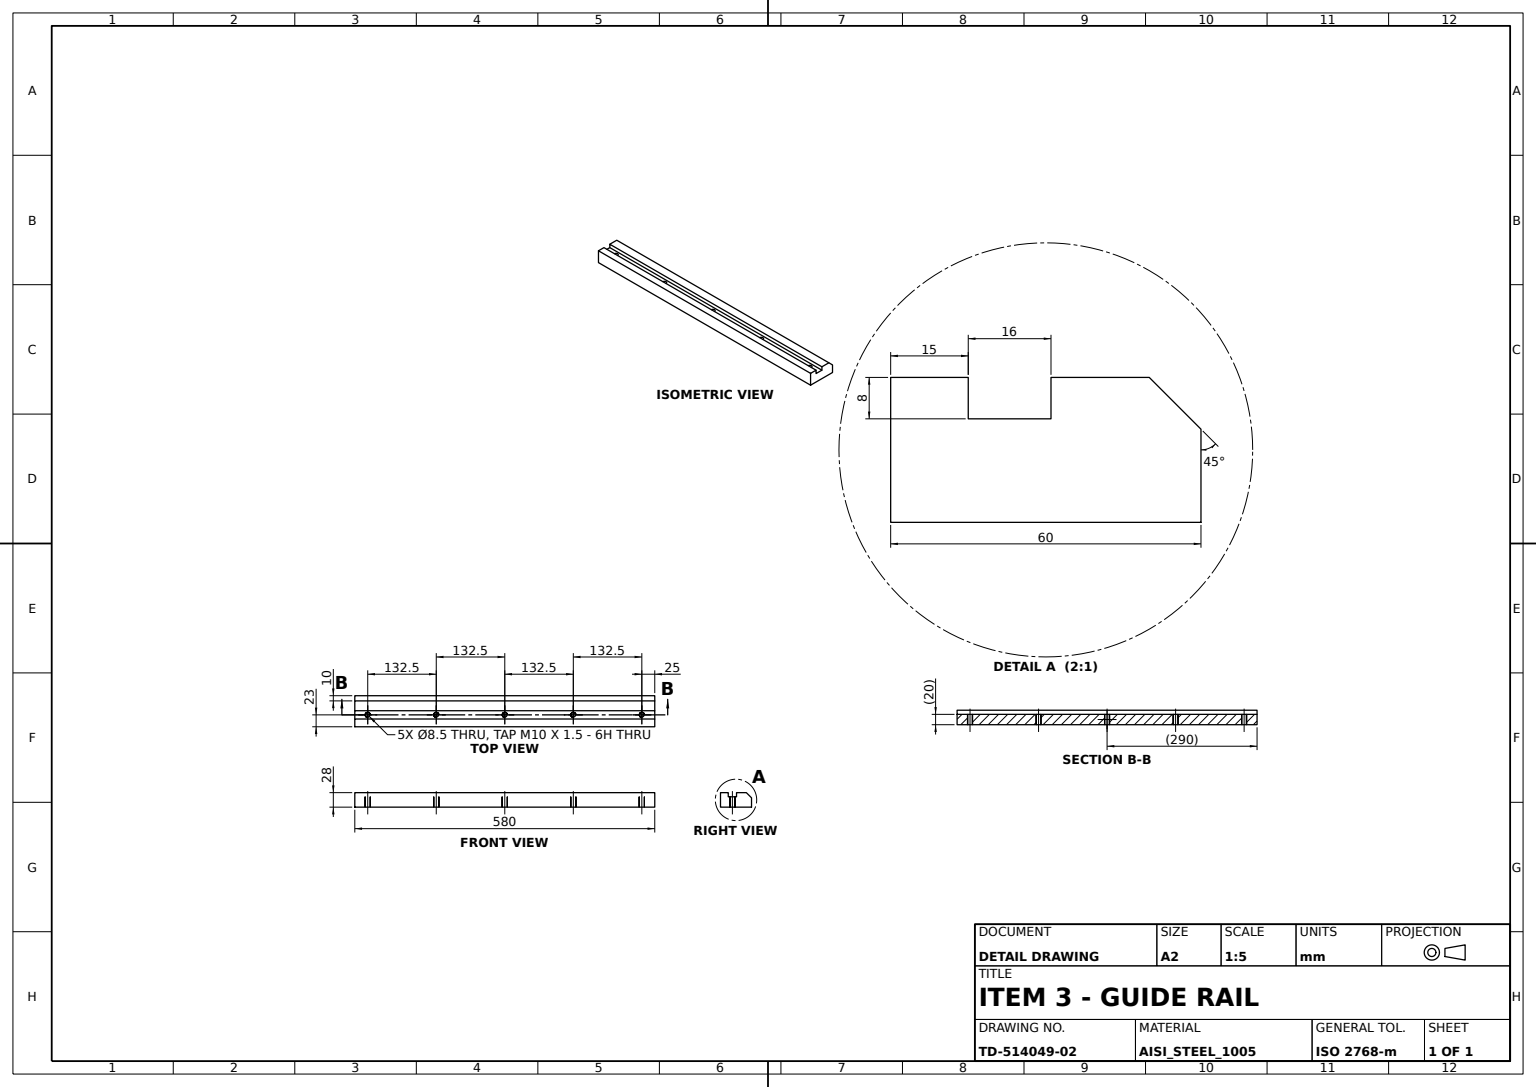
ISO-10303-21;
HEADER;
FILE_DESCRIPTION((''),'2;1');
FILE_NAME('','',(''),(''),'','','');
FILE_SCHEMA(('AUTOMOTIVE_DESIGN'));
ENDSEC;
DATA;
#1=APPLICATION_CONTEXT('');
#2=PRODUCT_CONTEXT('',#1,'mechanical');
#3=PRODUCT('','','',(#2));
#4=PRODUCT_DEFINITION_FORMATION('','',#3);
#5=PRODUCT_DEFINITION_CONTEXT('',#1,'design');
#6=PRODUCT_DEFINITION('','',#4,#5);
#7=PRODUCT_DEFINITION_SHAPE('','',#6);
#8=(LENGTH_UNIT()NAMED_UNIT(*)SI_UNIT(.MILLI.,.METRE.));
#9=(NAMED_UNIT(*)PLANE_ANGLE_UNIT()SI_UNIT($,.RADIAN.));
#10=(NAMED_UNIT(*)SI_UNIT($,.STERADIAN.)SOLID_ANGLE_UNIT());
#11=UNCERTAINTY_MEASURE_WITH_UNIT(LENGTH_MEASURE(0.005),#8,'distance_accuracy_value','');
#12=(GEOMETRIC_REPRESENTATION_CONTEXT(3)GLOBAL_UNCERTAINTY_ASSIGNED_CONTEXT((#11))GLOBAL_UNIT_ASSIGNED_CONTEXT((#8,#9,#10))REPRESENTATION_CONTEXT('',''));
#13=CARTESIAN_POINT('',(0.,32.75,265.));
#14=VERTEX_POINT('',#13);
#15=CARTESIAN_POINT('',(0.,37.,265.));
#16=DIRECTION('',(-1.,0.,0.));
#17=DIRECTION('',(0.,-1.,0.));
#18=AXIS2_PLACEMENT_3D('',#15,#16,#17);
#19=CIRCLE('',#18,4.25);
#20=EDGE_CURVE('',#14,#14,#19,.T.);
#21=ORIENTED_EDGE('',*,*,#20,.F.);
#22=EDGE_LOOP('',(#21));
#23=FACE_BOUND('',#22,.T.);
#24=CARTESIAN_POINT('',(-20.,41.25,265.));
#25=VERTEX_POINT('',#24);
#26=CARTESIAN_POINT('',(-20.,37.,265.));
#27=DIRECTION('',(1.,0.,0.));
#28=DIRECTION('',(0.,1.,0.));
#29=AXIS2_PLACEMENT_3D('',#26,#27,#28);
#30=CIRCLE('',#29,4.25);
#31=EDGE_CURVE('',#25,#25,#30,.T.);
#32=ORIENTED_EDGE('',*,*,#31,.F.);
#33=EDGE_LOOP('',(#32));
#34=FACE_BOUND('',#33,.T.);
#35=CYLINDRICAL_SURFACE('',#29,4.25);
#36=ADVANCED_FACE('',(#23,#34),#35,.F.);
#37=CARTESIAN_POINT('',(-20.,41.25,-132.5));
#38=VERTEX_POINT('',#37);
#39=CARTESIAN_POINT('',(-20.,37.,-132.5));
#40=AXIS2_PLACEMENT_3D('',#39,#27,#28);
#41=CIRCLE('',#40,4.25);
#42=EDGE_CURVE('',#38,#38,#41,.T.);
#43=ORIENTED_EDGE('',*,*,#42,.F.);
#44=EDGE_LOOP('',(#43));
#45=FACE_BOUND('',#44,.T.);
#46=CARTESIAN_POINT('',(0.,32.75,-132.5));
#47=VERTEX_POINT('',#46);
#48=CARTESIAN_POINT('',(0.,37.,-132.5));
#49=AXIS2_PLACEMENT_3D('',#48,#16,#17);
#50=CIRCLE('',#49,4.25);
#51=EDGE_CURVE('',#47,#47,#50,.T.);
#52=ORIENTED_EDGE('',*,*,#51,.F.);
#53=EDGE_LOOP('',(#52));
#54=FACE_BOUND('',#53,.T.);
#55=CYLINDRICAL_SURFACE('',#40,4.25);
#56=ADVANCED_FACE('',(#45,#54),#55,.F.);
#57=CARTESIAN_POINT('',(0.,60.,290.));
#58=VERTEX_POINT('',#57);
#59=CARTESIAN_POINT('',(-28.,60.,290.));
#60=VERTEX_POINT('',#59);
#61=VECTOR('',#16,1000.);
#62=LINE('',#57,#61);
#63=EDGE_CURVE('',#58,#60,#62,.T.);
#64=ORIENTED_EDGE('',*,*,#63,.F.);
#65=CARTESIAN_POINT('',(0.,60.,-290.));
#66=VERTEX_POINT('',#65);
#67=DIRECTION('',(0.,0.,-1.));
#68=VECTOR('',#67,1000.);
#69=LINE('',#57,#68);
#70=EDGE_CURVE('',#58,#66,#69,.T.);
#71=ORIENTED_EDGE('',*,*,#70,.T.);
#72=CARTESIAN_POINT('',(-28.,60.,-290.));
#73=VERTEX_POINT('',#72);
#74=LINE('',#65,#61);
#75=EDGE_CURVE('',#66,#73,#74,.T.);
#76=ORIENTED_EDGE('',*,*,#75,.T.);
#77=LINE('',#59,#68);
#78=EDGE_CURVE('',#60,#73,#77,.T.);
#79=ORIENTED_EDGE('',*,*,#78,.F.);
#80=EDGE_LOOP('',(#64,#71,#76,#79));
#81=FACE_BOUND('',#80,.T.);
#82=AXIS2_PLACEMENT_3D('',#57,#17,#27);
#83=PLANE('',#82);
#84=ADVANCED_FACE('',(#81),#83,.F.);
#85=CARTESIAN_POINT('',(-20.,29.,-290.));
#86=VERTEX_POINT('',#85);
#87=CARTESIAN_POINT('',(-28.,29.,-290.));
#88=VERTEX_POINT('',#87);
#89=LINE('',#85,#61);
#90=EDGE_CURVE('',#86,#88,#89,.T.);
#91=ORIENTED_EDGE('',*,*,#90,.T.);
#92=CARTESIAN_POINT('',(-28.,29.,290.));
#93=VERTEX_POINT('',#92);
#94=LINE('',#92,#68);
#95=EDGE_CURVE('',#93,#88,#94,.T.);
#96=ORIENTED_EDGE('',*,*,#95,.F.);
#97=CARTESIAN_POINT('',(-20.,29.,290.));
#98=VERTEX_POINT('',#97);
#99=LINE('',#97,#61);
#100=EDGE_CURVE('',#98,#93,#99,.T.);
#101=ORIENTED_EDGE('',*,*,#100,.F.);
#102=LINE('',#97,#68);
#103=EDGE_CURVE('',#98,#86,#102,.T.);
#104=ORIENTED_EDGE('',*,*,#103,.T.);
#105=EDGE_LOOP('',(#91,#96,#101,#104));
#106=FACE_BOUND('',#105,.T.);
#107=AXIS2_PLACEMENT_3D('',#97,#17,#27);
#108=PLANE('',#107);
#109=ADVANCED_FACE('',(#106),#108,.F.);
#110=CARTESIAN_POINT('',(0.,32.75,0.));
#111=VERTEX_POINT('',#110);
#112=CARTESIAN_POINT('',(0.,37.,0.));
#113=AXIS2_PLACEMENT_3D('',#112,#16,#17);
#114=CIRCLE('',#113,4.25);
#115=EDGE_CURVE('',#111,#111,#114,.T.);
#116=ORIENTED_EDGE('',*,*,#115,.F.);
#117=EDGE_LOOP('',(#116));
#118=FACE_BOUND('',#117,.T.);
#119=CARTESIAN_POINT('',(-20.,41.25,0.));
#120=VERTEX_POINT('',#119);
#121=CARTESIAN_POINT('',(-20.,37.,0.));
#122=AXIS2_PLACEMENT_3D('',#121,#27,#28);
#123=CIRCLE('',#122,4.25);
#124=EDGE_CURVE('',#120,#120,#123,.T.);
#125=ORIENTED_EDGE('',*,*,#124,.F.);
#126=EDGE_LOOP('',(#125));
#127=FACE_BOUND('',#126,.T.);
#128=CYLINDRICAL_SURFACE('',#122,4.25);
#129=ADVANCED_FACE('',(#118,#127),#128,.F.);
#130=ORIENTED_EDGE('',*,*,#115,.T.);
#131=EDGE_LOOP('',(#130));
#132=FACE_BOUND('',#131,.T.);
#133=CARTESIAN_POINT('',(0.,0.,290.));
#134=VERTEX_POINT('',#133);
#135=CARTESIAN_POINT('',(0.,0.,-290.));
#136=VERTEX_POINT('',#135);
#137=LINE('',#133,#68);
#138=EDGE_CURVE('',#134,#136,#137,.T.);
#139=ORIENTED_EDGE('',*,*,#138,.T.);
#140=VECTOR('',#28,1000.);
#141=LINE('',#135,#140);
#142=EDGE_CURVE('',#136,#66,#141,.T.);
#143=ORIENTED_EDGE('',*,*,#142,.T.);
#144=ORIENTED_EDGE('',*,*,#70,.F.);
#145=LINE('',#133,#140);
#146=EDGE_CURVE('',#134,#58,#145,.T.);
#147=ORIENTED_EDGE('',*,*,#146,.F.);
#148=EDGE_LOOP('',(#139,#143,#144,#147));
#149=FACE_BOUND('',#148,.T.);
#150=CARTESIAN_POINT('',(0.,32.75,132.5));
#151=VERTEX_POINT('',#150);
#152=CARTESIAN_POINT('',(0.,37.,132.5));
#153=AXIS2_PLACEMENT_3D('',#152,#16,#17);
#154=CIRCLE('',#153,4.25);
#155=EDGE_CURVE('',#151,#151,#154,.T.);
#156=ORIENTED_EDGE('',*,*,#155,.T.);
#157=EDGE_LOOP('',(#156));
#158=FACE_BOUND('',#157,.T.);
#159=ORIENTED_EDGE('',*,*,#51,.T.);
#160=EDGE_LOOP('',(#159));
#161=FACE_BOUND('',#160,.T.);
#162=CARTESIAN_POINT('',(0.,32.75,-265.));
#163=VERTEX_POINT('',#162);
#164=CARTESIAN_POINT('',(0.,37.,-265.));
#165=AXIS2_PLACEMENT_3D('',#164,#16,#17);
#166=CIRCLE('',#165,4.25);
#167=EDGE_CURVE('',#163,#163,#166,.T.);
#168=ORIENTED_EDGE('',*,*,#167,.T.);
#169=EDGE_LOOP('',(#168));
#170=FACE_BOUND('',#169,.T.);
#171=ORIENTED_EDGE('',*,*,#20,.T.);
#172=EDGE_LOOP('',(#171));
#173=FACE_BOUND('',#172,.T.);
#174=AXIS2_PLACEMENT_3D('',#133,#16,#17);
#175=PLANE('',#174);
#176=ADVANCED_FACE('',(#132,#149,#158,#161,#170,#173),#175,.F.);
#177=CARTESIAN_POINT('',(-20.,41.25,132.5));
#178=VERTEX_POINT('',#177);
#179=CARTESIAN_POINT('',(-20.,37.,132.5));
#180=AXIS2_PLACEMENT_3D('',#179,#27,#28);
#181=CIRCLE('',#180,4.25);
#182=EDGE_CURVE('',#178,#178,#181,.T.);
#183=ORIENTED_EDGE('',*,*,#182,.T.);
#184=EDGE_LOOP('',(#183));
#185=FACE_BOUND('',#184,.T.);
#186=ORIENTED_EDGE('',*,*,#124,.T.);
#187=EDGE_LOOP('',(#186));
#188=FACE_BOUND('',#187,.T.);
#189=ORIENTED_EDGE('',*,*,#103,.F.);
#190=CARTESIAN_POINT('',(-20.,45.,290.));
#191=VERTEX_POINT('',#190);
#192=VECTOR('',#17,1000.);
#193=LINE('',#190,#192);
#194=EDGE_CURVE('',#191,#98,#193,.T.);
#195=ORIENTED_EDGE('',*,*,#194,.F.);
#196=CARTESIAN_POINT('',(-20.,45.,-290.));
#197=VERTEX_POINT('',#196);
#198=LINE('',#190,#68);
#199=EDGE_CURVE('',#191,#197,#198,.T.);
#200=ORIENTED_EDGE('',*,*,#199,.T.);
#201=LINE('',#196,#192);
#202=EDGE_CURVE('',#197,#86,#201,.T.);
#203=ORIENTED_EDGE('',*,*,#202,.T.);
#204=EDGE_LOOP('',(#189,#195,#200,#203));
#205=FACE_BOUND('',#204,.T.);
#206=CARTESIAN_POINT('',(-20.,41.25,-265.));
#207=VERTEX_POINT('',#206);
#208=CARTESIAN_POINT('',(-20.,37.,-265.));
#209=AXIS2_PLACEMENT_3D('',#208,#27,#28);
#210=CIRCLE('',#209,4.25);
#211=EDGE_CURVE('',#207,#207,#210,.T.);
#212=ORIENTED_EDGE('',*,*,#211,.T.);
#213=EDGE_LOOP('',(#212));
#214=FACE_BOUND('',#213,.T.);
#215=ORIENTED_EDGE('',*,*,#31,.T.);
#216=EDGE_LOOP('',(#215));
#217=FACE_BOUND('',#216,.T.);
#218=ORIENTED_EDGE('',*,*,#42,.T.);
#219=EDGE_LOOP('',(#218));
#220=FACE_BOUND('',#219,.T.);
#221=AXIS2_PLACEMENT_3D('',#190,#27,#28);
#222=PLANE('',#221);
#223=ADVANCED_FACE('',(#185,#188,#205,#214,#217,#220),#222,.F.);
#224=ORIENTED_EDGE('',*,*,#155,.F.);
#225=EDGE_LOOP('',(#224));
#226=FACE_BOUND('',#225,.T.);
#227=ORIENTED_EDGE('',*,*,#182,.F.);
#228=EDGE_LOOP('',(#227));
#229=FACE_BOUND('',#228,.T.);
#230=CYLINDRICAL_SURFACE('',#180,4.25);
#231=ADVANCED_FACE('',(#226,#229),#230,.F.);
#232=ORIENTED_EDGE('',*,*,#167,.F.);
#233=EDGE_LOOP('',(#232));
#234=FACE_BOUND('',#233,.T.);
#235=ORIENTED_EDGE('',*,*,#211,.F.);
#236=EDGE_LOOP('',(#235));
#237=FACE_BOUND('',#236,.T.);
#238=CYLINDRICAL_SURFACE('',#209,4.25);
#239=ADVANCED_FACE('',(#234,#237),#238,.F.);
#240=CARTESIAN_POINT('',(-28.,45.,290.));
#241=VERTEX_POINT('',#240);
#242=LINE('',#59,#192);
#243=EDGE_CURVE('',#60,#241,#242,.T.);
#244=ORIENTED_EDGE('',*,*,#243,.T.);
#245=VECTOR('',#27,1000.);
#246=LINE('',#240,#245);
#247=EDGE_CURVE('',#241,#191,#246,.T.);
#248=ORIENTED_EDGE('',*,*,#247,.T.);
#249=ORIENTED_EDGE('',*,*,#194,.T.);
#250=ORIENTED_EDGE('',*,*,#100,.T.);
#251=CARTESIAN_POINT('',(-28.,10.,290.));
#252=VERTEX_POINT('',#251);
#253=LINE('',#92,#192);
#254=EDGE_CURVE('',#93,#252,#253,.T.);
#255=ORIENTED_EDGE('',*,*,#254,.T.);
#256=CARTESIAN_POINT('',(-18.,0.,290.));
#257=VERTEX_POINT('',#256);
#258=DIRECTION('',(0.707106781,-0.707106781,0.));
#259=VECTOR('',#258,1000.);
#260=LINE('',#251,#259);
#261=EDGE_CURVE('',#252,#257,#260,.T.);
#262=ORIENTED_EDGE('',*,*,#261,.T.);
#263=LINE('',#256,#245);
#264=EDGE_CURVE('',#257,#134,#263,.T.);
#265=ORIENTED_EDGE('',*,*,#264,.T.);
#266=ORIENTED_EDGE('',*,*,#146,.T.);
#267=ORIENTED_EDGE('',*,*,#63,.T.);
#268=EDGE_LOOP('',(#244,#248,#249,#250,#255,#262,#265,#266,#267));
#269=FACE_BOUND('',#268,.T.);
#270=DIRECTION('',(0.,0.,1.));
#271=AXIS2_PLACEMENT_3D('',#133,#270,#27);
#272=PLANE('',#271);
#273=ADVANCED_FACE('',(#269),#272,.T.);
#274=ORIENTED_EDGE('',*,*,#264,.F.);
#275=CARTESIAN_POINT('',(-18.,0.,-290.));
#276=VERTEX_POINT('',#275);
#277=LINE('',#256,#68);
#278=EDGE_CURVE('',#257,#276,#277,.T.);
#279=ORIENTED_EDGE('',*,*,#278,.T.);
#280=LINE('',#275,#245);
#281=EDGE_CURVE('',#276,#136,#280,.T.);
#282=ORIENTED_EDGE('',*,*,#281,.T.);
#283=ORIENTED_EDGE('',*,*,#138,.F.);
#284=EDGE_LOOP('',(#274,#279,#282,#283));
#285=FACE_BOUND('',#284,.T.);
#286=AXIS2_PLACEMENT_3D('',#256,#28,#270);
#287=PLANE('',#286);
#288=ADVANCED_FACE('',(#285),#287,.F.);
#289=ORIENTED_EDGE('',*,*,#261,.F.);
#290=CARTESIAN_POINT('',(-28.,10.,-290.));
#291=VERTEX_POINT('',#290);
#292=LINE('',#251,#68);
#293=EDGE_CURVE('',#252,#291,#292,.T.);
#294=ORIENTED_EDGE('',*,*,#293,.T.);
#295=LINE('',#290,#259);
#296=EDGE_CURVE('',#291,#276,#295,.T.);
#297=ORIENTED_EDGE('',*,*,#296,.T.);
#298=ORIENTED_EDGE('',*,*,#278,.F.);
#299=EDGE_LOOP('',(#289,#294,#297,#298));
#300=FACE_BOUND('',#299,.T.);
#301=DIRECTION('',(0.707106781,0.707106781,0.));
#302=DIRECTION('',(-0.707106781,0.707106781,0.));
#303=AXIS2_PLACEMENT_3D('',#251,#301,#302);
#304=PLANE('',#303);
#305=ADVANCED_FACE('',(#300),#304,.F.);
#306=CARTESIAN_POINT('',(-28.,45.,-290.));
#307=VERTEX_POINT('',#306);
#308=LINE('',#306,#245);
#309=EDGE_CURVE('',#307,#197,#308,.T.);
#310=ORIENTED_EDGE('',*,*,#309,.F.);
#311=LINE('',#72,#192);
#312=EDGE_CURVE('',#73,#307,#311,.T.);
#313=ORIENTED_EDGE('',*,*,#312,.F.);
#314=ORIENTED_EDGE('',*,*,#75,.F.);
#315=ORIENTED_EDGE('',*,*,#142,.F.);
#316=ORIENTED_EDGE('',*,*,#281,.F.);
#317=ORIENTED_EDGE('',*,*,#296,.F.);
#318=LINE('',#87,#192);
#319=EDGE_CURVE('',#88,#291,#318,.T.);
#320=ORIENTED_EDGE('',*,*,#319,.F.);
#321=ORIENTED_EDGE('',*,*,#90,.F.);
#322=ORIENTED_EDGE('',*,*,#202,.F.);
#323=EDGE_LOOP('',(#310,#313,#314,#315,#316,#317,#320,#321,#322));
#324=FACE_BOUND('',#323,.T.);
#325=AXIS2_PLACEMENT_3D('',#135,#270,#27);
#326=PLANE('',#325);
#327=ADVANCED_FACE('',(#324),#326,.F.);
#328=ORIENTED_EDGE('',*,*,#243,.F.);
#329=ORIENTED_EDGE('',*,*,#78,.T.);
#330=ORIENTED_EDGE('',*,*,#312,.T.);
#331=LINE('',#240,#68);
#332=EDGE_CURVE('',#241,#307,#331,.T.);
#333=ORIENTED_EDGE('',*,*,#332,.F.);
#334=EDGE_LOOP('',(#328,#329,#330,#333));
#335=FACE_BOUND('',#334,.T.);
#336=AXIS2_PLACEMENT_3D('',#59,#27,#28);
#337=PLANE('',#336);
#338=ADVANCED_FACE('',(#335),#337,.F.);
#339=ORIENTED_EDGE('',*,*,#199,.F.);
#340=ORIENTED_EDGE('',*,*,#247,.F.);
#341=ORIENTED_EDGE('',*,*,#332,.T.);
#342=ORIENTED_EDGE('',*,*,#309,.T.);
#343=EDGE_LOOP('',(#339,#340,#341,#342));
#344=FACE_BOUND('',#343,.T.);
#345=AXIS2_PLACEMENT_3D('',#240,#28,#270);
#346=PLANE('',#345);
#347=ADVANCED_FACE('',(#344),#346,.F.);
#348=ORIENTED_EDGE('',*,*,#254,.F.);
#349=ORIENTED_EDGE('',*,*,#95,.T.);
#350=ORIENTED_EDGE('',*,*,#319,.T.);
#351=ORIENTED_EDGE('',*,*,#293,.F.);
#352=EDGE_LOOP('',(#348,#349,#350,#351));
#353=FACE_BOUND('',#352,.T.);
#354=AXIS2_PLACEMENT_3D('',#92,#27,#28);
#355=PLANE('',#354);
#356=ADVANCED_FACE('',(#353),#355,.F.);
#357=CLOSED_SHELL('',(#36,#56,#84,#109,#129,#176,#223,#231,#239,#273,#288,#305,#327,#338,#347,#356));
#358=MANIFOLD_SOLID_BREP('',#357);
#359=ADVANCED_BREP_SHAPE_REPRESENTATION('',(#358),#12);
#360=SHAPE_DEFINITION_REPRESENTATION(#7,#359);
ENDSEC;
END-ISO-10303-21;
